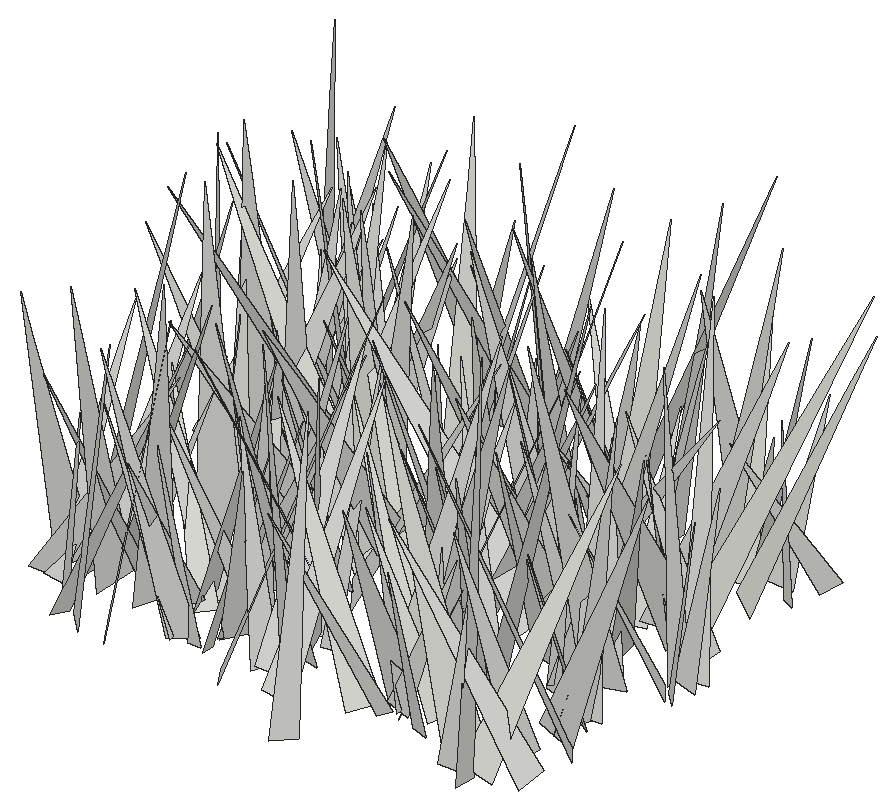
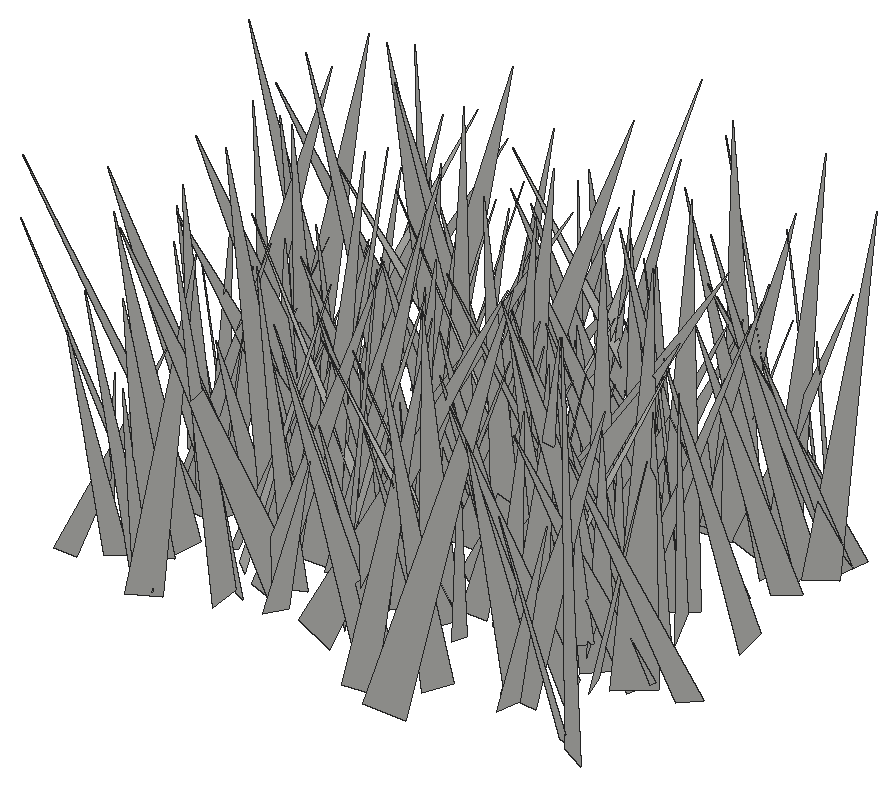
# SketchUp Ruby script. Lengths in inches.
U = 1.inch
M = Sketchup.active_model
def pt(a) = Geom::Point3d.new(a.map { |v| v * U })
def face(e, loops, mat)
  f = e.add_face(loops[0].map { |a| pt(a) })
  loops[1..].each { |l| e.add_face(l.map { |a| pt(a) }).erase! }
  f.material = f.back_material = mat if mat
  f
end
# faces: each face lists its corners as indices into pts; further lists are holes
def faces(e, pts, list, mat = nil) = list.each { |f| face(e, (f[0].is_a?(Array) ? f : [f]).map { |l| l.map { |i| pts[i] } }, mat) }
# xy, xz, yz: faces in a plane at the given z, y or x. An outline is a flat list of corners, or four numbers for a rectangle; further outlines are holes
def ring(l) = l.size == 4 ? [[l[0], l[1]], [l[2], l[1]], [l[2], l[3]], [l[0], l[3]]] : l.each_slice(2).to_a
def flat(e, list, mat, &to3) = list.each { |f| face(e, (f[0].is_a?(Array) ? f : [f]).map { |l| ring(l).map { |u, v| to3.(u, v) } }, mat) }
def xy(e, z, list, mat = nil) = flat(e, list, mat) { |x, y| [x, y, z] }
def xz(e, y, list, mat = nil) = flat(e, list, mat) { |x, z| [x, y, z] }
def yz(e, x, list, mat = nil) = flat(e, list, mat) { |y, z| [x, y, z] }
def lines(e, pts, list) = list.each { |a, b| e.add_line(pt(pts[a]), pt(pts[b])) }
# prism: a flat outline (further loops are holes) pulled along v
def prism(e, loops, v, mat = nil)
  f = face(e, loops, mat); d = Geom::Vector3d.new(v.map { |x| x * U })
  f.pushpull(f.normal.samedirection?(d) ? d.length : -d.length)
end
def box(e, o, s, mat = nil) = prism(e, [[o, [o[0] + s[0], o[1], o[2]], [o[0] + s[0], o[1] + s[1], o[2]], [o[0], o[1] + s[1], o[2]]]], [0, 0, s[2]], mat)
def at(x, y, z, deg = 0) = Geom::Transformation.translation(pt([x, y, z])) * Geom::Transformation.rotation(ORIGIN, Z_AXIS, deg.degrees)
def axes(o, x, y, z) = Geom::Transformation.new([*x, 0, *y, 0, *z, 0, *pt(o).to_a, 1])
def part(name) = M.definitions.add(name)
# library, detail: a bought-in or finely detailed component or shape, given as its bounding box
def library(name, o, s) = part(name).tap { |d| box(d.entities, o, s) }
def detail(e, o, s) = box(e.add_group.entities, o, s)
def put(e, d, t, mat = nil) = e.add_instance(d, t).tap { |i| i.material = mat if mat }
def group(e, t, mat = nil) = e.add_group.tap { |g| g.transformation = t; g.material = mat if mat }.entities
root = M.entities
c1 = part("fur_instance\#9")
p = [[0.8125,0,1.79],[0.67,-0.02,1.48],[0,-0.11,0],[0,0.11,0]]
faces(c1.entities,p,[[0,1,2,3]])
put(root,c1,axes([150.06,251.15,-27.1],[-5.67085,1.89535,1.35099],[1.57668,5.74544,-1.44226],[1.71219,0.98676,5.80265]))
put(root,c1,axes([155.92,253.25,-27.1],[0.94774,-3.5048,1.15841],[-3.67796,-0.79512,0.60341],[0.31324,1.26803,3.58018]))
put(root,c1,axes([140.08,253.44,-27.1],[6.22111,3.48137,1.76986],[3.77865,-6.20685,-1.07301],[-0.98698,-1.81924,7.04775]))
put(root,c1,axes([158.84,254.34,-27.1],[-5.67147,0.82087,0.04901],[0.80443,5.46726,1.5178],[-0.17066,-1.50898,5.5259]))
put(root,c1,axes([138.85,253.22,-27.1],[4.00395,3.96639,1.91354],[4.25291,-4.1539,-0.28869],[-1.14309,-1.56151,5.62855]))
put(root,c1,axes([153.53,254.58,-27.1],[-0.97443,-3.66118,0.75209],[-3.71136,1.03977,0.25308],[0.44234,0.6588,3.78017]))
put(root,c1,axes([142.61,254.66,-27.1],[0.82361,-5.861,1.93807],[-5.93962,-1.28507,-1.3621],[-1.68178,1.66825,5.75972]))
put(root,c1,axes([151.41,256.34,-27.1],[5.27025,-2.47106,0.85487],[-2.00329,-5.05203,-2.25305],[-1.68041,-1.72721,5.36707]))
put(root,c1,axes([157.63,255.57,-27.1],[-4.78026,1.17069,2.19317],[1.89155,4.79719,1.56216],[1.61324,-2.15588,4.66702]))
put(root,c1,axes([155.46,254.74,-27.1],[3.76435,-5.16952,3.38659],[-5.24976,-4.76711,-1.44149],[-3.26082,1.70703,6.23028]))
put(root,c1,axes([137.65,254.11,-27.1],[-2.04031,-2.94511,1.87891],[-3.25881,2.38849,0.20512],[1.25863,1.41005,3.57693]))
put(root,c1,axes([138.14,256.35,-27.1],[6.98441,-2.34407,2.00985],[-1.86712,-7.16517,-1.86827],[-2.45928,-1.21733,7.12645]))
put(root,c1,axes([151.6875,254.9,-27.1],[-1.12844,-4.06047,0.83548],[-3.60524,0.5338,-2.27512],[-2.04639,1.29864,3.54749]))
put(root,c1,axes([141.48,256.68,-27.1],[3.03189,-3.59681,0.02756],[-3.43565,-2.90654,-1.37057],[-1.06494,-0.8632,4.50011]))
put(root,c1,axes([157.08,252.74,-27.1],[-7.37531,-1.40171,2.74866],[-2.16749,7.42249,-2.03071],[2.19589,2.61858,7.22747]))
put(root,c1,axes([143.98,255.93,-27.1],[3.85722,-2.97975,0.1804],[-2.96484,-3.85827,-0.33622],[-0.3481,-0.15623,4.86251]))
put(root,c1,axes([142.22,254.75,-27.1],[-4.50006,-1.01814,0.39176],[-1.03948,4.50642,-0.22865],[0.331,0.31016,4.60813]))
put(root,c1,axes([147.51,258.19,-27.1],[-4.65731,-6.85842,0.0184],[-6.74044,4.58127,1.51895],[1.26677,-0.83835,8.14992]))
put(root,c1,axes([136.05,256.73,-27.1],[5.91516,-3.3432,1.65321],[-2.9566,-6.09276,-1.74243],[-2.27346,-0.77492,6.56735]))
put(root,c1,axes([143.23,254.56,-27.1],[0.75971,3.71481,1.88794],[3.89435,-1.31575,1.02184],[-1.48263,-1.55251,3.65142]))
put(root,c1,axes([146.2,254.92,-27.1],[-4.24357,2.27798,1.78244],[2.54082,4.44811,0.36434],[1.38223,-1.18292,4.80254]))
put(root,c1,axes([140.07,256.2,-27.1],[6.97183,-3.45055,1.53762],[-3.37643,-7.13932,-0.71191],[-1.69419,0.0288,7.74635]))
put(root,c1,axes([148.16,253.84,-27.1],[-6.10428,-1.79449,1.71008],[-2.20054,6.01533,-1.54278],[1.14113,2.0006,6.1727]))
put(root,c1,axes([139.66,256.67,-27.1],[-1.20375,-5.21342,0.24756],[-5.17288,1.15789,-0.76855],[-0.69453,0.4118,5.2951]))
put(root,c1,axes([151.89,255.4,-27.1],[0.78956,-4.05986,1.16414],[-3.93825,-0.27989,1.69498],[1.52574,1.37851,3.77266]))
put(root,c1,axes([150.81,254.78,-27.1],[-4.45803,3.98436,0.74293],[4.03358,4.25341,1.39275],[-0.39655,-1.52789,5.81458]))
put(root,c1,axes([137.97,253.4,-27.1],[5.78446,0.51407,0.77192],[0.25637,-5.57234,1.78981],[-0.89129,1.73346,5.52457]))
put(root,c1,axes([147.09,256.15,-27.1],[-2.90211,-6.23156,1.67253],[-6.44447,2.71044,-1.08359],[-0.31368,1.96803,6.78825]))
put(root,c1,axes([156.99,253.51,-27.1],[0.07577,6.70614,0.84141],[6.48392,0.16538,-1.90197],[1.90764,-0.82847,6.43122]))
put(root,c1,axes([153.46,255.8125,-27.1],[-3.79672,1.89832,0.59417],[1.98792,3.66583,0.99077],[0.06937,-1.15319,4.1276]))
put(root,c1,axes([147.94,253.375,-27.1],[0.187,6.43803,0.46404],[6.40843,-0.12967,-0.78342],[0.77175,-0.48321,6.39292]))
put(root,c1,axes([135.7,255.36,-27.1],[4.06898,-3.86093,0.67624],[-3.71406,-3.48612,2.44405],[1.25293,2.20473,5.04877]))
put(root,c1,axes([158.81,256.73,-27.1],[-5.4011,-4.4458,0.12135],[-4.40164,5.31613,-1.14717],[-0.63674,0.96192,6.9008]))
put(root,c1,axes([143.81,254.6,-27.1],[3.84083,1.33111,0.88578],[1.09907,-3.87194,1.0529],[-1.16125,0.73803,3.92622]))
put(root,c1,axes([152,255.625,-27.1],[-4.7779,-0.84592,1.0787],[-0.97294,4.84801,-0.50762],[0.9657,0.69908,4.82558]))
put(root,c1,axes([145.41,253.28,-27.1],[6.47525,4.61232,0.40047],[4.47579,-6.41261,1.48613],[-1.18373,0.98374,7.80985]))
put(root,c1,axes([152.64,256.84,-27.1],[1.6475,-3.20979,0.84583],[-3.31321,-1.64761,0.20101],[-0.20196,0.8456,3.6023]))
put(root,c1,axes([157.54,257.38,-27.1],[1.03631,-6.95808,1.71035],[-6.57848,-0.23906,3.0134],[2.83968,1.98547,6.35675]))
put(root,c1,axes([146.55,257.31,-27.1],[5.52429,1.58059,2.16664],[1.98524,-5.74559,-0.8703],[-1.80317,-1.48335,5.67966]))
put(root,c1,axes([137.67,257.47,-27.1],[7.30646,0.41261,0.41525],[0.46932,-7.23653,-1.06747],[-0.34987,-1.09065,7.23983]))
put(root,c1,axes([143.98,257.26,-27.1],[-0.35504,-4.51922,1.36303],[-4.31721,-0.2418,-1.92625],[-1.90863,1.3876,4.10353]))
put(root,c1,axes([146.66,254.6875,-27.1],[-1.23708,6.4323,0.84499],[6.38548,1.35924,-0.99849],[1.14637,-0.62994,6.47363]))
put(root,c1,axes([141.63,257.15,-27.1],[5.98361,0.11352,0.76596],[0.13466,-6.02993,-0.15823],[-0.76252,-0.17402,5.9826]))
put(root,c1,axes([136.29,255.22,-27.1],[0.97806,5.36378,0.25201],[5.36787,-0.98334,0.09641],[-0.14015,-0.23057,5.45137]))
put(root,c1,axes([143.35,258.02,-27.1],[4.53528,-3.04969,1.17101],[-3.07507,-4.66168,-0.23091],[-1.10265,0.45689,5.46041]))
put(root,c1,axes([149.2,256.92,-27.1],[-4.27231,-1.94809,0.06255],[-1.87913,4.07681,-1.37844],[-0.51754,1.27912,4.48861]))
put(root,c1,axes([157.16,258,-27.1],[4.10425,1.09153,0.3293],[1.14011,-3.92312,-1.20584],[0.00571,-1.24998,4.07214]))
put(root,c1,axes([151.17,256.32,-27.1],[1.96643,7.28816,1.86053],[7.47956,-1.69089,-1.28167],[0.79683,-2.11408,7.43918]))
put(root,c1,axes([143.74,255.58,-27.1],[3.9731,1.20771,1.01378],[0.70264,-3.81635,1.79266],[-1.41159,1.49959,3.74573]))
put(root,c1,axes([151.63,257.01,-27.1],[-3.45745,4.3845,0.64107],[4.38114,3.2607,1.32749],[-0.66366,-1.31634,5.42361]))
put(root,c1,axes([152.15,259.57,-27.1],[-0.85203,-5.57664,0.61964],[-5.3803,0.98986,1.51043],[1.59225,0.36067,5.43539]))
put(root,c1,axes([150.91,258.63,-27.1],[6.79044,-4.4332,0.71146],[-4.48312,-6.76549,0.63187],[-0.24718,0.91888,8.0848]))
put(root,c1,axes([141.97,256.74,-27.1],[-2.66965,3.73747,0.14274],[3.69986,2.61324,0.77338],[-0.54785,-0.56423,4.52743]))
put(root,c1,axes([141.83,257.65,-27.1],[-5.56985,2.38046,0.65327],[2.45077,5.52546,0.76123],[0.29505,-0.95874,6.00918]))
put(root,c1,axes([152.17,255.27,-27.1],[5.76242,3.50846,0.12226],[3.39302,-5.62636,1.53663],[-0.90093,1.2508,6.56914]))
put(root,c1,axes([157.83,258.61,-27.1],[-2.17535,-3.01047,0.60266],[-3.06621,2.16789,-0.23847],[0.15643,0.62897,3.70651]))
put(root,c1,axes([152.35,259.97,-27.1],[-3.97091,-3.72473,0.66515],[-3.58252,4.01146,1.07602],[1.21718,-0.34456,5.33703]))
put(root,c1,axes([136.98,256.42,-27.1],[7.21368,2.51232,2.17903],[2.05011,-7.45745,1.81123],[-2.61859,1.08246,7.42081]))
put(root,c1,axes([146.46,257.95,-27.1],[-0.50007,3.75556,1.02909],[3.87876,0.38868,0.46638],[-0.34425,-1.07612,3.75989]))
put(root,c1,axes([147.2,262.72,-27.1],[4.97759,-6.71856,0.2944],[-6.18791,-4.7191,-3.07278],[-2.63353,-1.61035,7.77647]))
put(root,c1,axes([142.9,256.89,-27.1],[1.96135,3.70682,0.36248],[3.45553,-1.96392,1.38604],[-1.38968,0.34826,3.95807]))
put(root,c1,axes([149.18,261.19,-27.1],[7.15666,-2.1147,0.99823],[-1.83229,-7.06792,-1.83669],[-1.45298,-1.50292,7.233]))
put(root,c1,axes([157.6875,258.72,-27.1],[5.90361,-0.69248,2.28384],[-0.937,-6.27702,0.51884],[-2.19488,0.81708,5.9214]))
put(root,c1,axes([150.68,261.49,-27.1],[-1.15105,-5.30671,0.17],[-5.09537,1.15297,1.49093],[1.49242,-0.15644,5.22142]))
put(root,c1,axes([142.31,259.48,-27.1],[-3.28529,-1.60429,1.12724],[-1.66632,3.44368,0.04462],[1.03333,0.45264,3.6558]))
put(root,c1,axes([156.66,261.3,-27.1],[1.61042,-7.88282,1.5376],[-7.97737,-1.75156,-0.62458],[-0.92985,1.37466,8.02136]))
put(root,c1,axes([142.35,258.57,-27.1],[5.41003,-2.25588,0.78895],[-2.38957,-5.13634,1.69936],[-0.03699,1.87321,5.60977]))
put(root,c1,axes([136.34,258.32,-27.1],[-0.72846,5.64896,1.65026],[5.62241,1.15927,-1.48642],[1.73859,-1.38206,5.49837]))
put(root,c1,axes([153.78,261.51,-27.1],[-0.77388,-5.77446,0.46112],[-5.72229,0.83441,0.84559],[0.90132,0.33953,5.76439]))
put(root,c1,axes([153.49,258.86,-27.1],[8.05424,1.38868,1.7961],[1.29513,-8.24767,0.56905],[-1.86468,0.26973,8.15325]))
put(root,c1,axes([147.1875,257.33,-27.1],[1.91748,5.33638,0.31642],[5.10909,-1.9283,1.55969],[-1.57297,0.24194,5.4517]))
put(root,c1,axes([150.89,261.25,-27.1],[-5.52316,-3.7636,0.965],[-3.71814,5.60658,0.58551],[1.12752,0.05244,6.65787]))
put(root,c1,axes([137.57,259.08,-27.1],[2.54826,3.20038,0.28055],[3.20908,-2.5526,-0.02947],[-0.15164,-0.23787,4.09087]))
put(root,c1,axes([138.67,261.76,-27.1],[5.1556,-5.75467,2.21602],[-5.90961,-5.43588,-0.36737],[-1.76168,1.39363,7.71761]))
put(root,c1,axes([145.36,260.9,-27.1],[5.77692,4.11347,0.10405],[3.90568,-5.42514,-2.37018],[1.29504,-1.98782,6.68399]))
put(root,c1,axes([158.59,262.33,-27.1],[-3.47143,-2.84551,0.09651],[-2.81271,3.45107,0.57956],[0.4415,-0.38766,4.45106]))
put(root,c1,axes([155.74,263.28,-27.1],[6.93671,-0.62868,0.23505],[-0.51232,-6.5363,-2.3628],[-0.4336,-2.33453,6.55213]))
put(root,c1,axes([157.57,259.125,-27.1],[1.24745,7.40868,1.63783],[7.39275,-1.56046,1.42803],[-1.70827,-1.34297,7.376]))
put(root,c1,axes([155.36,261.83,-27.1],[0.47741,-4.86513,1.33169],[-4.92648,-0.73691,-0.92606],[-1.08291,1.20759,4.79999]))
put(root,c1,axes([144.97,261.13,-27.1],[0.7235,3.49331,2.20248],[3.65755,-1.58024,1.30491],[-1.91742,-1.69623,3.32022]))
put(root,c1,axes([142.81,259.35,-27.1],[5.29795,0.17393,1.896],[-0.4687,-5.31448,1.7972],[-1.84537,1.84915,4.98684]))
put(root,c1,axes([141.83,263.91,-27.1],[2.44843,-5.51273,0.60157],[-4.8536,-2.44839,-2.68234],[-2.6823,-0.60174,5.40279]))
put(root,c1,axes([138.97,260.97,-27.1],[5.52113,3.74347,2.2115],[4.00437,-5.77059,-0.2291],[-1.6939,-1.44011,6.66663]))
put(root,c1,axes([155.43,259.87,-27.1],[2.35955,4.93164,1.36493],[4.86886,-2.62618,1.07189],[-1.57426,-0.73054,5.36093]))
put(root,c1,axes([152.09,264.41,-27.1],[4.15216,-5.25606,0.30062],[-4.95254,-4.0295,-2.04756],[-1.78575,-1.04593,6.37763]))
put(root,c1,axes([151.65,260.72,-27.1],[-4.9618,2.41645,1.1014],[2.44275,5.06865,-0.11597],[1.04177,-0.37582,5.51772]))
put(root,c1,axes([149.36,260.875,-27.1],[-0.86303,4.80618,1.97762],[4.83833,1.47497,-1.47315],[1.8976,-1.57489,4.65553]))
put(root,c1,axes([155.25,261.94,-27.1],[-0.48209,-3.49328,1.24378],[-3.69826,0.54426,0.09516],[0.26993,1.21786,3.5251]))
put(root,c1,axes([157.15,265.59,-27.1],[4.52461,-6.7861,0.00105],[-6.53347,-4.35651,-2.20405],[-1.83437,-1.22185,7.85273]))
put(root,c1,axes([149.17,260.37,-27.1],[-2.13966,5.92839,0.3544],[5.56639,1.87053,2.31645],[-2.07043,-1.09766,5.86157]))
put(root,c1,axes([152.4375,264.36,-27.1],[-3.66849,-5.82093,1.22872],[-5.44278,3.86666,2.06783],[2.40191,-0.1285,6.56241]))
put(root,c1,axes([151.82,263.59,-27.1],[-7.78216,2.50032,0.23977],[2.4235,7.26917,2.85602],[-0.66011,-2.78901,7.65877]))
put(root,c1,axes([139.53,263.59,-27.1],[-6.5147,0.26004,1.16019],[0.55336,6.38259,1.67669],[1.05235,-1.74639,6.3006]))
put(root,c1,axes([156.18,262.09,-27.1],[-2.69115,3.5868,1.84623],[3.86426,2.92918,-0.05799],[1.15809,-1.43902,4.48375]))
put(root,c1,axes([159.03,262.1,-27.1],[-2.22453,-2.28888,1.93607],[-2.6411,2.63697,0.08289],[1.41842,1.32035,3.19071]))
put(root,c1,axes([144.74,263.6,-27.1],[4.88048,-6.02987,2.56967],[-6.14977,-5.32095,-0.80587],[-2.26779,1.4525,7.7155]))
put(root,c1,axes([158.85,263.12,-27.1],[0.22976,-4.49295,1.68417],[-4.67204,0.17468,1.10336],[1.09322,1.69077,4.36142]))
put(root,c1,axes([144.38,265.2,-27.1],[-2.23996,-8.03771,0.28468],[-7.44594,1.96073,-3.22749],[-3.04036,1.11981,7.69451]))
put(root,c1,axes([135.1,261.95,-27.1],[6.05583,0.88682,1.38397],[0.67013,-6.15634,1.01257],[-1.50092,0.82941,6.03608]))
put(root,c1,axes([155.43,260.57,-27.1],[7.73551,0.03019,2.73159],[-1.01366,-7.58581,2.95441],[-2.53672,3.12332,7.14916]))
put(root,c1,axes([144.4375,264.15,-27.1],[0.04247,-7.07988,2.41623],[-7.48051,-0.06275,-0.05238],[-0.06984,2.41579,7.07981]))
put(root,c1,axes([149.96,262.82,-27.1],[5.54197,-0.978,0.47716],[-1.05474,-5.437,1.10644],[-0.26776,1.17482,5.51777]))
put(root,c1,axes([139.78,264.8125,-27.1],[6.66168,-2.88093,2.18206],[-2.80757,-7.00677,-0.67958],[-2.27567,0.211,7.22605]))
put(root,c1,axes([158.44,263.3125,-27.1],[-5.81537,-0.03657,1.70774],[-0.23888,6.01751,-0.6846],[1.69135,0.72416,5.77505]))
put(root,c1,axes([145.93,264.57,-27.1],[-2.3451,-4.39084,0.71964],[-4.31416,2.04482,-1.58228],[-1.08875,1.35503,4.71968]))
put(root,c1,axes([144.76,263.09,-27.1],[-4.02573,7.19257,0.41274],[6.48293,3.4104,3.80141],[-3.14246,-2.17854,7.31361]))
put(root,c1,axes([157.27,264.48,-27.1],[-3.81411,-2.18756,1.38745],[-2.30966,3.98998,-0.05835],[1.17299,0.74331,4.39652]))
put(root,c1,axes([151.97,263.91,-27.1],[4.55,-4.60588,0.41001],[-4.16176,-3.82822,3.1795],[2.01545,2.49305,5.6398]))
put(root,c1,axes([142.47,261.37,-27.1],[2.76635,7.35948,0.05567],[7.35952,-2.76581,-0.07342],[0.04914,-0.07794,7.86188]))
put(root,c1,axes([143.23,265.42,-27.1],[0.67729,-7.55263,2.0847],[-7.70125,-0.25666,1.57216],[1.44182,2.17688,7.41817]))
put(root,c1,axes([158.24,265.22,-27.1],[-5.1344,0.67452,1.09766],[0.89094,5.11676,1.02317],[0.93062,-1.17714,5.07643]))
put(root,c1,axes([144.15,266.5,-27.1],[0.26999,-5.16111,0.17986],[-5.16087,-0.27616,-0.17741],[-0.18667,0.17024,5.16512]))
put(root,c1,axes([137.7,262.68,-27.1],[-6.50203,-1.48304,1.94789],[-2.15091,6.10063,-2.53495],[1.1693,2.97539,6.16846]))
put(root,c1,axes([138.15,263.4,-27.1],[0.38602,5.6901,1.15392],[5.67114,-0.61727,1.14668],[-1.24374,-1.04858,5.58671]))
put(root,c1,axes([137.91,266.1,-27.1],[3.24769,-2.54753,0.32293],[-2.51539,-3.26077,-0.4265],[-0.51676,-0.13836,4.10555]))
put(root,c1,axes([150.83,267.07,-27.1],[-0.69616,-7.71222,1.47846],[-7.81205,0.83092,0.65597],[0.79755,1.40715,7.71575]))
put(root,c1,axes([152.71,267.49,-27.1],[3.43107,-2.8474,0.0502],[-2.64084,-3.2106,-1.6126],[-1.06592,-1.21113,4.15686]))
put(root,c1,axes([138.87,264.2,-27.1],[-2.71022,2.78687,0.60598],[2.7235,2.77712,-0.59105],[0.8464,-0.01233,3.84222]))
put(root,c1,axes([153.89,268.05,-27.1],[-4.54437,-2.07997,0.71062],[-1.49312,4.11891,2.50752],[1.61302,-2.04715,4.32318]))
put(root,c1,axes([149.75,266.92,-27.1],[-6.14349,2.42883,3.06477],[3.31416,6.26335,1.67969],[2.07568,-2.81172,6.38908]))
put(root,c1,axes([151.89,266.2,-27.1],[4.55769,0.07164,0.01251],[0.0727,-4.46545,-0.91231],[0.00209,-0.91239,4.46602]))
put(root,c1,axes([158.87,263.6,-27.1],[0.5538,7.06628,1.29605],[7.05626,-0.7792,1.23321],[-1.34954,-1.17443,6.97985]))
put(root,c1,axes([148.31,265.11,-27.1],[4.95013,-1.23925,0.4471],[-1.29852,-4.88303,0.8422],[-0.22245,0.9272,5.03291]))
put(root,c1,axes([147.76,268,-27.1],[0.04578,-6.29285,0.19538],[-6.21134,-0.07706,-1.02644],[-1.02831,0.18529,6.20874]))
put(root,c1,axes([136.24,267.2,-27.1],[5.79688,-5.3049,1.7816],[-5.31494,-6.02201,-0.63769],[-1.75142,0.71643,7.83193]))
put(root,c1,axes([148.92,265.37,-27.1],[6.16739,3.42449,0.19717],[3.4017,-6.05394,-1.25736],[0.441,-1.19388,6.94138]))
put(root,c1,axes([148.3,264.84,-27.1],[2.54415,2.86578,1.34064],[2.68524,-2.86561,1.02977],[-1.67317,-0.2414,3.6912]))
put(root,c1,axes([147.15,265.48,-27.1],[-5.93557,-1.05009,0.32847],[-1.08922,5.86272,-0.94003],[0.15548,0.98355,5.95399]))
put(root,c1,axes([146.39,267.71,-27.1],[5.5268,-1.95543,1.04999],[-1.67194,-5.52102,-1.48142],[-1.45972,-1.07995,5.67227]))
put(root,c1,axes([137.53,264.87,-27.1],[-2.26569,5.88907,2.62757],[5.5866,3.18358,-2.31806],[3.22106,-1.37923,5.86866]))
put(root,c1,axes([141.54,267.07,-27.1],[-5.94217,-4.1756,0.21971],[-4.13273,5.80684,-1.41225],[-0.63601,1.27993,7.12394]))
put(root,c1,axes([155.44,266.02,-27.1],[4.70932,-5.02611,1.74089],[-5.27526,-4.11549,2.38842],[0.68127,2.87596,6.46026]))
put(root,c1,axes([153.48,265.78,-27.1],[-0.77106,7.66776,2.67234],[8.04873,1.0768,-0.76736],[1.07416,-2.56446,7.66813]))
put(root,c1,axes([142.625,265.18,-27.1],[-6.42625,-2.81034,1.42452],[-3.14557,5.90814,-2.53441],[0.18076,2.90169,6.53999]))
put(root,c1,axes([154.64,265.5,-27.1],[-1.99149,3.68652,0.84504],[3.6319,2.13053,-0.73532],[1.05538,-0.37542,4.12502]))
put(root,c1,axes([138.19,266.69,-27.1],[-3.99726,2.72851,1.81883],[2.89094,4.28575,-0.07581],[1.5477,-0.9584,4.83912]))
put(root,c1,axes([152.8,268.96,-27.1],[-3.72414,-4.2026,0.59605],[-4.10843,3.76818,0.89886],[1.06672,-0.15915,5.54285]))
put(root,c1,axes([138.09,266.95,-27.1],[3.39124,-4.48702,2.29298],[-4.9912,-3.37077,0.78574],[-0.69206,2.32297,5.56924]))
put(root,c1,axes([145.99,265.37,-27.1],[3.94824,4.29759,0.4959],[4.2386,-3.97723,0.72087],[-0.86569,0.12707,5.79122]))
put(root,c1,axes([147.875,267.72,-27.1],[-2.80028,2.24736,2.49663],[2.73085,3.4158,-0.01176],[1.95607,-1.55147,3.59055]))
put(root,c1,axes([141.38,266.72,-27.1],[-0.70822,-5.57958,3.0516],[-6.3293,0.31925,-0.88519],[-0.61961,3.1164,5.55425]))
put(root,c1,axes([149.0625,268.66,-27.1],[-4.24041,-4.62675,0.86788],[-4.65391,4.29598,0.16351],[0.70788,0.52807,6.27385]))
put(root,c1,axes([138.03,265.67,-27.1],[7.54644,-1.30772,2.23251],[-1.88035,-7.50036,1.96263],[-1.77721,2.38276,7.40318]))
put(root,c1,axes([143.09,265.93,-27.1],[-5.60196,1.71083,0.59088],[1.59688,5.57635,-1.00614],[0.85208,0.79713,5.77032]))
put(root,c1,axes([140.47,266.23,-27.1],[0.3651,6.79595,1.75212],[7.01816,-0.34958,-0.10649],[0.01583,-1.75528,6.80491]))
put(root,c1,axes([141.18,267.02,-27.1],[4.31663,-3.25233,1.38409],[-3.53279,-4.03972,1.52536],[-0.11299,2.05661,5.185]))
put(root,c1,axes([137.58,267.85,-27.1],[-4.67685,-1.64881,1.07356],[-1.71505,4.77313,-0.14071],[0.96421,0.49258,4.95698]))
put(root,c1,axes([140.96,267.55,-27.1],[-6.02179,2.8816,2.13168],[3.11245,6.27078,0.31555],[1.77772,-1.21792,6.66828]))
put(root,c1,axes([140.3125,268.18,-27.1],[5.34451,-3.5502,0.35957],[-3.55754,-5.25077,1.03462],[0.27778,1.05952,6.33224]))
put(root,c1,axes([143.46,268.2,-27.1],[3.51099,-0.42801,1.09439],[-0.295,-3.65871,-0.48452],[-1.13748,-0.37227,3.50364]))
put(root,c1,axes([136.15,266.89,-27.1],[3.23121,-4.00646,1.7311],[-4.24322,-2.37965,2.41277],[1.02152,2.78831,4.54653]))
put(root,c1,axes([156.83,266.06,-27.1],[0.48963,4.22721,0.04806],[3.94805,-0.47454,1.51627],[-1.51146,0.12987,3.97618]))
put(root,c1,axes([138.74,266.9375,-27.1],[-2.41477,3.3901,0.55663],[3.41153,2.44646,-0.10002],[0.40504,-0.3947,4.161]))
put(root,c1,axes([134.17,266.6,-27.1],[-0.28996,5.60424,1.15409],[5.32871,0.68543,-1.98963],[2.08431,-0.97272,5.24719]))
put(root,c1,axes([150.3,269.04,-27.1],[-0.32261,-5.78503,1.74562],[-5.69921,0.87225,1.8374],[2.00818,1.5461,5.49497]))
put(root,c1,axes([150.92,269.99,-27.1],[-1.61608,-6.86234,1.14057],[-6.89566,1.42577,-1.19223],[-0.91789,1.37106,6.94853]))
put(root,c1,axes([156.31,266.93,-27.1],[3.48936,7.09192,0.65775],[6.9322,-3.21357,-2.12629],[1.63479,-1.51038,7.61247]))
put(root,c1,axes([147.73,271.17,-27.1],[-1.57704,-7.74459,0.50786],[-7.45096,1.36569,-2.31124],[-2.17253,0.93802,7.55804]))
put(root,c1,axes([144.63,267.89,-27.1],[-6.2785,3.87073,1.88034],[3.7817,6.55006,-0.85632],[2.05354,-0.22787,7.32591]))
put(root,c1,axes([147.68,269.62,-27.1],[-5.07554,-4.81191,2.50581],[-5.17107,5.32884,-0.24106],[1.64121,1.90882,6.98981]))
put(root,c1,axes([138.97,270.41,-27.1],[1.01091,-5.94061,2.30759],[-6.04054,-1.63799,-1.57056],[-2.03168,1.91413,5.81775]))
put(root,c1,axes([156.77,269.125,-27.1],[3.72746,5.46093,0.78491],[5.42353,-3.45332,-1.72965],[1.01153,-1.60767,6.38153]))
put(root,c1,axes([144.35,268.88,-27.1],[4.3038,1.80689,1.01933],[1.67441,-4.41138,0.75005],[-1.22483,0.31842,4.60705]))
put(root,c1,axes([144.78,266.51,-27.1],[5.37795,5.75,0.47067],[5.40496,-5.24661,2.33794],[-2.01755,1.27162,7.51791]))
put(root,c1,axes([158.48,272.02,-27.1],[2.70067,-3.13661,0.88183],[-2.51329,-2.73437,-2.02883],[-2.07348,-0.77102,3.60774]))
put(root,c1,axes([146.38,269.36,-27.1],[5.52496,2.9641,0.73245],[3.00682,-5.54515,-0.24054],[-0.53047,-0.55942,6.26523]))
put(root,c1,axes([155.25,269.33,-27.1],[6.61649,-1.70465,2.3436],[-2.13195,-6.81989,1.0584],[-1.96294,1.66119,6.75008]))
put(root,c1,axes([145.32,270.36,-27.1],[4.26673,-0.51352,0.23406],[-0.5171,-4.27238,0.05285],[-0.22604,0.08052,4.29719]))
put(root,c1,axes([137.9,268.7,-27.1],[6.18202,1.83786,0.77531],[1.68935,-6.16651,1.14736],[-1.06062,0.8903,6.34654]))
put(root,c1,axes([151.6,270.66,-27.1],[3.4231,3.63538,1.50249],[3.93251,-3.11512,-1.42212],[0.09387,-2.06666,4.78656]))
put(root,c1,axes([157.96,270.19,-27.1],[1.56672,2.93333,1.48069],[3.11219,-1.85095,0.37383],[-1.05412,-1.105,3.30444]))
put(root,c1,axes([143.98,273.34,-27.1],[-0.13701,-6.93499,0.01519],[-6.899,0.13785,0.70555],[0.70571,0.00117,6.90036]))
put(root,c1,axes([142.22,274.05,-27.1],[1.01288,-8.11783,0.06805],[-8.08119,-1.01477,-0.77093],[-0.77341,-0.02823,8.14437]))
put(root,c1,axes([141.82,271.46,-27.1],[5.79925,-1.98106,0.58125],[-1.98372,-5.82701,-0.06806],[-0.57211,0.1232,6.12791]))
put(root,c1,axes([139.27,269.84,-27.1],[4.10356,-2.98524,2.70877],[-3.77942,-4.1935,1.10399],[-1.40181,2.56732,4.95298]))
put(root,c1,axes([154.3,272.72,-27.1],[4.71186,-4.25626,1.34995],[-4.06485,-4.9009,-1.26409],[-1.848,-0.07223,6.22249]))
put(root,c1,axes([156.91,271.04,-27.1],[-0.57371,3.97778,1.97621],[4.19128,1.14438,-1.08668],[1.47014,-1.71025,3.86924]))
put(root,c1,axes([155.93,270.97,-27.1],[5.31059,0.52385,1.16283],[0.52648,-5.43598,0.04446],[-1.16164,-0.06886,5.33618]))
put(root,c1,axes([155.65,270.28,-27.1],[-2.00411,5.21831,1.67163],[5.38658,2.20263,-0.41796],[1.00489,-1.39973,5.57427]))
put(root,c1,axes([150.6,269.3,-27.1],[8.13769,0.92636,1.08085],[0.65484,-8.00564,1.93114],[-1.26395,1.81658,7.95932]))
put(root,c1,axes([151.89,271.04,-27.1],[7.00703,0.38351,2.14023],[0.30488,-7.32356,0.31416],[-2.15283,0.21111,7.01048]))
put(root,c1,axes([139.01,270.95,-27.1],[-4.50468,1.1443,0.55643],[1.12699,4.53841,-0.20945],[0.5907,0.0676,4.64302]))
put(root,c1,axes([154.46,272.5625,-27.1],[0.84418,-3.62493,0.18375],[-3.45271,-0.74384,1.18829],[1.11924,0.43944,3.52714]))
put(root,c1,axes([149.88,270.7,-27.1],[-3.84574,2.31871,0.01808],[2.31862,3.84577,-0.02193],[0.02681,0.00945,4.49062]))
put(root,c1,axes([145.96,270.42,-27.1],[6.16496,0.12051,1.82007],[-0.27856,-6.27765,1.3592],[-1.80266,1.38221,6.01447]))
put(root,c1,axes([134.89,272.42,-27.1],[4.42565,6.01002,3.52258],[6.87552,-4.43985,-1.06317],[-1.12079,-3.50468,7.38759]))
put(root,c1,axes([135.84,271.7,-27.1],[2.6257,3.60497,0.95618],[3.72031,-2.44904,-0.98281],[0.26337,-1.34567,4.35019]))
